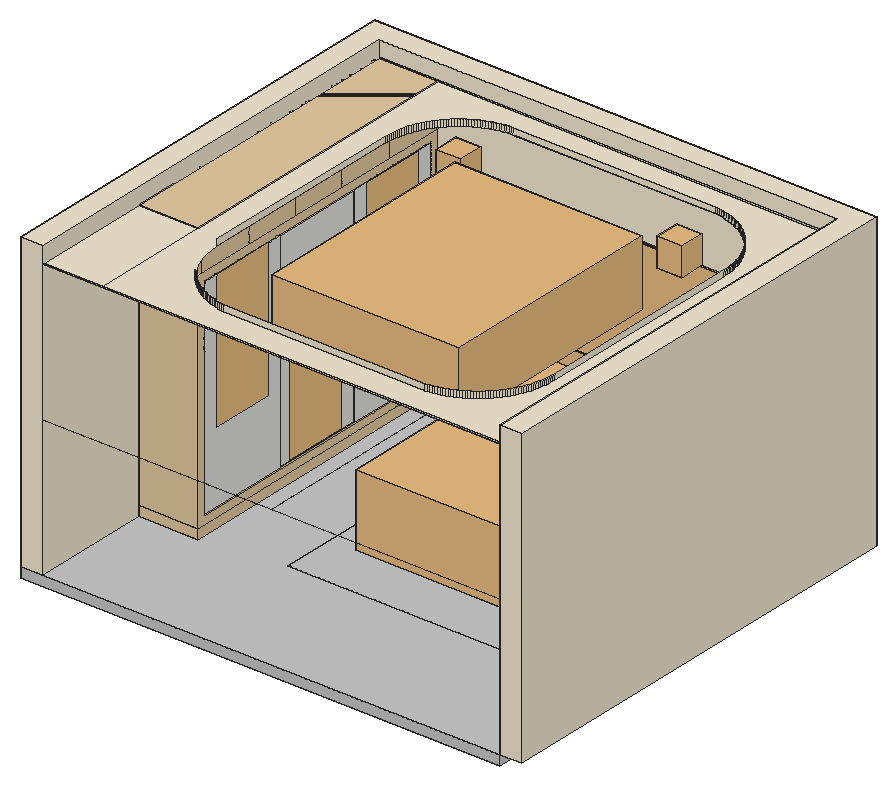
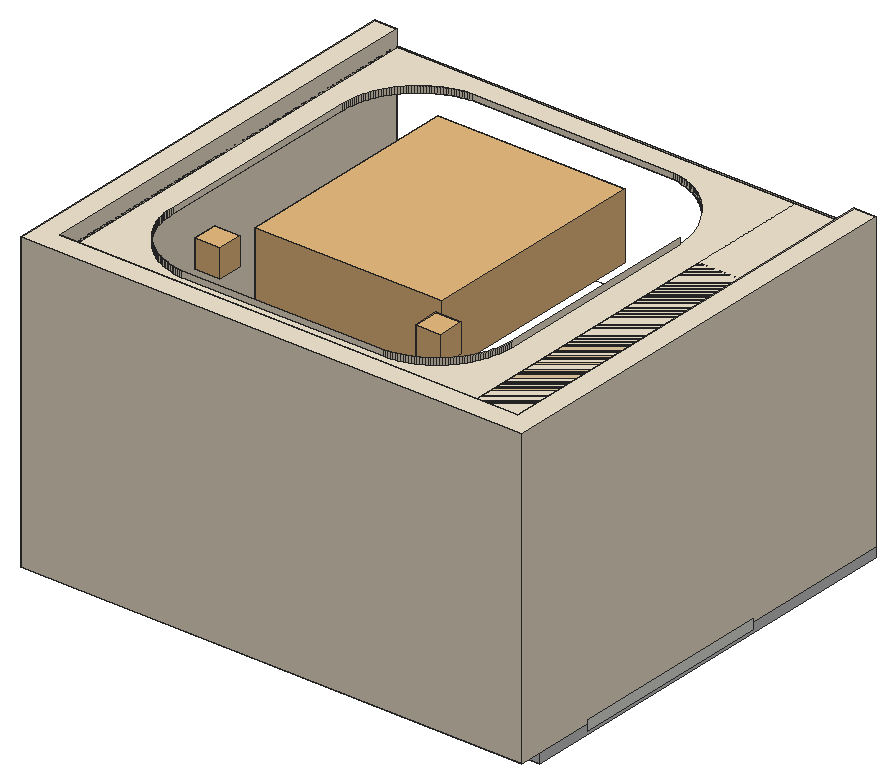
# SketchUp Ruby script. Lengths in inches.
U = 1.inch
M = Sketchup.active_model
def pt(a) = Geom::Point3d.new(a.map { |v| v * U })
def face(e, loops, mat)
  f = e.add_face(loops[0].map { |a| pt(a) })
  loops[1..].each { |l| e.add_face(l.map { |a| pt(a) }).erase! }
  f.material = f.back_material = mat if mat
  f
end
# faces: each face lists its corners as indices into pts; further lists are holes
def faces(e, pts, list, mat = nil) = list.each { |f| face(e, (f[0].is_a?(Array) ? f : [f]).map { |l| l.map { |i| pts[i] } }, mat) }
# xy, xz, yz: faces in a plane at the given z, y or x. An outline is a flat list of corners, or four numbers for a rectangle; further outlines are holes
def ring(l) = l.size == 4 ? [[l[0], l[1]], [l[2], l[1]], [l[2], l[3]], [l[0], l[3]]] : l.each_slice(2).to_a
def flat(e, list, mat, &to3) = list.each { |f| face(e, (f[0].is_a?(Array) ? f : [f]).map { |l| ring(l).map { |u, v| to3.(u, v) } }, mat) }
def xy(e, z, list, mat = nil) = flat(e, list, mat) { |x, y| [x, y, z] }
def xz(e, y, list, mat = nil) = flat(e, list, mat) { |x, z| [x, y, z] }
def yz(e, x, list, mat = nil) = flat(e, list, mat) { |y, z| [x, y, z] }
def lines(e, pts, list) = list.each { |a, b| e.add_line(pt(pts[a]), pt(pts[b])) }
# prism: a flat outline (further loops are holes) pulled along v
def prism(e, loops, v, mat = nil)
  f = face(e, loops, mat); d = Geom::Vector3d.new(v.map { |x| x * U })
  f.pushpull(f.normal.samedirection?(d) ? d.length : -d.length)
end
def box(e, o, s, mat = nil) = prism(e, [[o, [o[0] + s[0], o[1], o[2]], [o[0] + s[0], o[1] + s[1], o[2]], [o[0], o[1] + s[1], o[2]]]], [0, 0, s[2]], mat)
def at(x, y, z, deg = 0) = Geom::Transformation.translation(pt([x, y, z])) * Geom::Transformation.rotation(ORIGIN, Z_AXIS, deg.degrees)
def axes(o, x, y, z) = Geom::Transformation.new([*x, 0, *y, 0, *z, 0, *pt(o).to_a, 1])
def part(name) = M.definitions.add(name)
# library, detail: a bought-in or finely detailed component or shape, given as its bounding box
def library(name, o, s) = part(name).tap { |d| box(d.entities, o, s) }
def detail(e, o, s) = box(e.add_group.entities, o, s)
def put(e, d, t, mat = nil) = e.add_instance(d, t).tap { |i| i.material = mat if mat }
def group(e, t, mat = nil) = e.add_group.tap { |g| g.transformation = t; g.material = mat if mat }.entities
root = M.entities
M.materials.add("0961 AP 7892 PALE IVORY").color = [243, 232, 209]
M.materials.add("0962 AP 9878 Bamboo Straw-N").color = [228, 203, 161]
M.materials.add("Acquerello Marble (TJ07TT)").color = [202, 201, 200]
M.materials.add("Generic").color = [255, 255, 255]
M.materials.add("Kit Kat Speckle_ Stack (OYOLJ5)").color = [227, 224, 217]
M.materials.add("The Belden Brick Company Dapple Gray Matt None Modular (3-5-").color = [200, 200, 200]
c1 = library("ceiling fan",[0,0,0],[76.25,93.13,30.02])
c2 = part("fan")
p = [[217.527,-902.72,540.318],[217.529,-902.72,540.318],[217.529,-902.72,541.354],[217.527,-902.72,541.354]]
lines(c2.entities,p,[[0,1],[2,3]])
put(c2.entities,c1,at(256.45,-350.9,679.41))
c3 = library("Side Table",[0,-0.77,-1.18],[23.62,18.49,23.93])
c4 = library("Group\#4",[-0.5,-1.92,0],[127,2.42,36])
c5 = library("Group\#18",[-0.5,-0.5,0],[151,1.71,48])
c6 = part("Group105\#1")
p = [[0,0,0],[0,0,-46.23],[-14.28,0,-46.23],[93,-56.66,0],[-93,-56.66,0],[93,56.66,0],
  [93,0,0],[-93,56.66,0],[14.28,0,-46.23],[-93,0,0],[0,0,-74.83]]
lines(c6.entities,p,[[0,1],[1,2],[3,4],[5,6],[7,5],[1,8],[9,0],[0,6],[8,10],[4,9],[6,3],[2,10],
  [9,7]])
c7 = part("Rectangle Light\#1")
put(c7.entities,c6,at(0,0,0))
c8 = library("Bed 001",[-37.84,-46.07,0],[75.19,90.39,37.01])
c9 = library("Group\#5",[-0.5,-0.74,0],[30,1.24,80])
c10 = part("Group8\#1")
xy(c10.entities,7,[[-26.93,80.42,-2.93,81.13],[-26.93,109.26,-2.93,109.97],[-26.93,138.1,-2.93,138.81]])
xy(c10.entities,42.65,[[-26.93,51.9375,-2.93,80.42],[-26.93,81.13,-2.93,109.26],[-26.93,109.97,-2.93,138.1],[-26.93,138.81,-2.93,167.29]])
xy(c10.entities,43.35,[[-26.93,51.9375,-2.93,80.78],[-26.93,80.78,-2.93,109.26],[-26.93,109.97,-2.93,138.45],[-26.93,138.45,-2.93,167.29]])
xy(c10.entities,93,[[-26.93,109.26,-2.93,109.97]])
xz(c10.entities,51.9375,[[-26.93,42.65,-2.93,43.35]])
xz(c10.entities,80.42,[[-26.93,7,-2.93,42.65]])
xz(c10.entities,81.13,[[-26.93,7,-2.93,42.65]])
xz(c10.entities,109.26,[[-26.93,7,-2.93,42.65],[-26.93,43.35,-2.93,93]])
xz(c10.entities,109.97,[[-26.93,7,-2.93,42.65],[-26.93,43.35,-2.93,93]])
xz(c10.entities,138.1,[[-26.93,7,-2.93,42.65]])
xz(c10.entities,138.81,[[-26.93,7,-2.93,42.65]])
xz(c10.entities,167.29,[[-26.93,42.65,-2.93,43.35]])
yz(c10.entities,-26.93,[[80.42,7,80.42,42.65,80.78,43,81.13,42.65,81.13,7],[109.26,7,109.26,42.65,109.61,43,109.97,42.65,109.97,7],[138.1,7,138.1,42.65,138.45,43,138.81,42.65,138.81,7],[51.9375,42.65,51.9375,43.35,80.78,43.35,80.78,43,80.42,42.65],[81.13,42.65,80.78,43,80.78,43.35,109.26,43.35,109.61,43,109.26,42.65],
  [109.97,42.65,109.61,43,109.97,43.35,138.45,43.35,138.45,43,138.1,42.65],[138.81,42.65,138.45,43,138.45,43.35,167.29,43.35,167.29,42.65],[109.61,43,109.26,43.35,109.26,93,109.97,93,109.97,43.35]])
yz(c10.entities,-2.93,[[80.42,7,81.13,7,81.13,42.65,80.78,43,80.42,42.65],[109.26,7,109.97,7,109.97,42.65,109.61,43,109.26,42.65],[138.1,7,138.81,7,138.81,42.65,138.45,43,138.1,42.65],[51.9375,42.65,80.42,42.65,80.78,43,80.78,43.35,51.9375,43.35],[81.13,42.65,109.26,42.65,109.61,43,109.26,43.35,80.78,43.35,80.78,43],
  [109.97,42.65,138.1,42.65,138.45,43,138.45,43.35,109.97,43.35,109.61,43],[138.81,42.65,167.29,42.65,167.29,43.35,138.45,43.35,138.45,43],[109.61,43,109.97,43.35,109.97,93,109.26,93,109.26,43.35]])
c11 = part("Group\#11")
box(c11.entities,[0,0,0],[0.71,37.98,84.58])
c12 = part("Group\#21")
box(c12.entities,[0,0,-0.71],[23.77,15.3125,0.71])
c13 = part("Group16\#1")
xy(c13.entities,96,[[-26.22,74.37,-0.64,75.08],[-26.22,98.16,-2.22,98.87],[-26.22,121.95,-2.22,122.65],[-26.22,145.73,-2.22,146.44]])
xy(c13.entities,111.3125,[[-26.22,74.37,-0.64,75.08],[-26.22,98.16,-2.22,98.87],[-26.22,121.95,-2.22,122.65],[-26.22,145.73,-2.22,146.44]])
xz(c13.entities,74.37,[[-26.22,96,-0.64,111.3125]])
xz(c13.entities,75.08,[[-26.22,96,-0.64,111.3125]])
xz(c13.entities,98.16,[[-26.22,96,-2.22,111.3125]])
xz(c13.entities,98.87,[[-26.22,96,-2.22,111.3125]])
xz(c13.entities,121.95,[[-26.22,96,-2.22,111.3125]])
xz(c13.entities,122.65,[[-26.22,96,-2.22,111.3125]])
xz(c13.entities,145.73,[[-26.22,96,-2.22,111.3125]])
xz(c13.entities,146.44,[[-26.22,96,-2.22,111.3125]])
yz(c13.entities,-26.22,[[74.37,96,75.08,111.3125],[98.16,96,98.87,111.3125],[121.95,96,122.65,111.3125],[145.73,96,146.44,111.3125]])
yz(c13.entities,-2.22,[[98.16,96,98.87,111.3125],[121.95,96,122.65,111.3125],[145.73,96,146.44,111.3125]])
yz(c13.entities,-0.64,[[74.37,96,75.08,111.3125]])
c14 = library("plafonjera+p5",[99.06,48.1875,1.61],[10.2,10.2,11.38])
xy(root,7,[[12.07,51.9375,34.66,138.45],[34.66,51.9375,36.07,51.9375,36.07,167.29,35.36,167.29,35.36,138.45,34.66,138.45],[12.07,138.45,34.66,167.29],[34.66,138.45,35.36,167.29]])
xy(root,7.71,[[34.66,52.65,35.36,166.58]])
xy(root,7.71,[[35.36,52.65,36.07,166.58]],"0962 AP 9878 Bamboo Straw-N")
xy(root,43,[[12.07,138.45,35.36,167.29]])
xy(root,92.29,[[34.66,52.65,35.36,166.58],[35.36,52.65,36.07,166.58]])
xy(root,93,[[12.07,51.9375,34.66,167.29],[34.66,51.9375,36.07,167.29]])
xy(root,96,[[12.07,48.9375,36.07,170.29]])
xy(root,113.3125,[[12,0,36,171],[[36,0,198,171],[76.2,12,158,12,158.91,12.1,159.8125,12.23,160.71,12.39,161.61,12.57,162.5,12.78,163.38,13.02,164.26,13.28,165.13,13.57,165.99,13.88,166.84,14.22,167.68,14.58,168.51,14.97,169.32,15.38,170.13,15.82,170.92,16.28,171.7,16.76,172.46,17.27,173.21,17.79,173.9375,18.34,174.65,18.91,175.35,19.5,176.03,20.11,176.69,20.74,177.34,21.39,177.96,22.0625,178.5625,22.75,179.15,23.45,179.71,24.18,180.25,24.91,180.77,25.67,181.27,26.43,181.74,27.22,182.19,28.01,182.62,28.82,183.02,29.64,183.4,30.47,183.75,31.32,184.08,32.17,184.39,33.03,184.66,33.91,184.92,34.78,185.14,35.67,185.34,36.5625,185.52,37.46,185.66,38.36,185.78,39.27,185.88,40.18,185.95,41.09,185.99,42.01,186,42.92,186,129,185.99,129.9,185.95,130.81,185.88,131.71,185.78,132.6,185.66,133.5,185.51,134.39,185.34,135.28,185.14,136.16,184.91,137.03,184.65,137.9,184.375,138.76,184.07,139.61,183.74,140.45,183.38,141.28,183,142.1,182.59,142.9,182.16,143.7,181.71,144.48,181.23,145.25,180.73,146,180.21,146.74,179.67,147.46,179.1,148.16,178.52,148.85,177.91,149.52,177.29,150.17,176.64,150.8,175.98,151.41,175.29,152.01,174.59,152.58,173.88,153.125,173.15,153.65,172.4,154.16,171.63,154.64,170.86,155.1,170.07,155.54,169.26,155.95,168.45,156.34,167.62,156.71,166.78,157.04,165.9375,157.36,165.08,157.65,164.22,157.91,163.34,158.14,162.47,158.35,161.58,158.54,160.69,158.69,159.8,158.82,158.9,158.92,158,159,76.2,159,75.3,158.93,74.39,158.83,73.5,158.71,72.6,158.56,71.71,158.38,70.83,158.17,69.95,157.94,69.08,157.6875,68.22,157.4,67.37,157.09,66.52,156.76,65.69,156.4,64.87,156.01,64.0625,155.6,63.27,155.17,62.48,154.71,61.71,154.23,60.96,153.72,60.22,153.19,59.5,152.64,58.8,152.07,58.11,151.48,57.4375,150.87,56.79,150.24,56.16,149.59,55.55,148.92,54.96,148.23,54.39,147.52,53.84,146.8,53.3125,146.06,52.81,145.31,52.33,144.54,51.87,143.75,51.4375,142.96,51.03,142.15,50.64,141.32,50.28,140.49,49.95,139.65,49.64,138.8,49.36,137.93,49.1,137.0625,48.875,136.1875,48.67,135.3,48.49,134.41,48.34,133.52,48.22,132.62,48.125,131.72,48.06,130.8125,48.01,129.91,48,129,48,43.85,48.01,42.92,48.06,41.99,48.12,41.0625,48.22,40.14,48.34,39.22,48.49,38.3,48.66,37.38,48.86,36.48,49.09,35.57,49.34,34.68,49.62,33.79,49.92,32.91,50.25,32.04,50.61,31.18,50.99,30.33,51.39,29.5,51.82,28.67,52.27,27.86,52.75,27.06,53.24,26.27,53.76,25.5,54.31,24.75,54.87,24.01,55.46,23.29,56.0625,22.58,56.69,21.89,57.34,21.22,58,20.57,58.6875,19.94,59.39,19.33,60.11,18.74,60.84,18.18,61.6,17.63,62.36,17.1,63.15,16.6,63.94,16.12,64.75,15.67,65.58,15.23,66.41,14.82,67.26,14.44,68.12,14.08,68.98,13.75,69.86,13.4375,70.75,13.15,71.64,12.9,72.54,12.66,73.45,12.46,74.36,12.28,75.28,12.125]]],"0961 AP 7892 PALE IVORY")
xz(root,0,[[12,113.3125,198,113.78]],"0961 AP 7892 PALE IVORY")
xz(root,12,[[76.2,113.3125,158,115.78]],"0961 AP 7892 PALE IVORY")
xz(root,48.9375,[[12.07,4,36.07,96]],"0962 AP 9878 Bamboo Straw-N")
xz(root,51.9375,[[12.07,7,34.66,93],[34.66,7,36.07,93]])
xz(root,52.65,[[34.66,7.71,35.36,92.29],[35.36,7.71,36.07,92.29]])
xz(root,138.45,[[12.07,7,35.36,43]])
xz(root,159,[[76.2,113.3125,158,115.78]],"0961 AP 7892 PALE IVORY")
xz(root,166.58,[[34.66,7.71,35.36,92.29],[35.36,7.71,36.07,92.29]])
xz(root,167.29,[[12.07,7,34.66,43],[34.66,7,35.36,43],[35.36,7,36.07,7,36.07,93,34.66,93,34.66,43,35.36,43],[12.07,43,34.66,93]])
xz(root,170.29,[[12.07,4,36.07,96]])
xz(root,171,[[12,113.3125,198,113.78]],"0961 AP 7892 PALE IVORY")
yz(root,12,[[0,113.3125,171,113.78]],"0961 AP 7892 PALE IVORY")
yz(root,12.07,[[[48.9375,4,170.29,96],[51.9375,7,167.29,93]],[51.9375,7,80.78,43],[80.78,7,109.61,43],[109.61,7,138.45,43],[51.9375,43,109.61,93],
  [109.61,43,167.29,93]])
yz(root,34.66,[[[51.9375,7,167.29,93],[52.65,7.71,166.58,92.29]]])
yz(root,35.36,[[138.45,7,167.29,7,167.29,43,166.58,43,166.58,7.71,138.45,7.71],[138.45,7.71,166.58,43]])
yz(root,36.07,[[[48.9375,4,170.29,96],[51.9375,7,167.29,93]],[[51.9375,7,167.29,93],[52.65,7.71,166.58,92.29]]],"0962 AP 9878 Bamboo Straw-N")
yz(root,48,[[43.85,113.3125,129,115.78]],"0961 AP 7892 PALE IVORY")
yz(root,186,[[42.92,113.3125,129,115.78]],"0961 AP 7892 PALE IVORY")
yz(root,198,[[0,113.3125,171,113.78]],"0961 AP 7892 PALE IVORY")
p = [[76.2,12,113.3125],[75.28,12.125,113.3125],[75.28,12.125,115.78],[76.2,12,115.78],[158.91,12.1,113.3125],[158,12,113.3125],
  [158,12,115.78],[158.91,12.1,115.78],[74.36,12.28,113.3125],[74.36,12.28,115.78],[159.8125,12.23,113.3125],[159.8125,12.23,115.78],
  [160.71,12.39,113.3125],[160.71,12.39,115.78],[73.45,12.46,113.3125],[73.45,12.46,115.78],[161.61,12.57,113.3125],[161.61,12.57,115.78],
  [72.54,12.66,113.3125],[72.54,12.66,115.78],[162.5,12.78,113.3125],[162.5,12.78,115.78],[71.64,12.9,113.3125],[71.64,12.9,115.78],
  [163.38,13.02,113.3125],[163.38,13.02,115.78],[70.75,13.15,113.3125],[70.75,13.15,115.78],[164.26,13.28,113.3125],[164.26,13.28,115.78],
  [69.86,13.4375,113.3125],[69.86,13.4375,115.78],[165.13,13.57,113.3125],[165.13,13.57,115.78],[68.98,13.75,113.3125],[68.98,13.75,115.78],
  [165.99,13.88,113.3125],[165.99,13.88,115.78],[68.12,14.08,113.3125],[68.12,14.08,115.78],[166.84,14.22,113.3125],[166.84,14.22,115.78],
  [67.26,14.44,113.3125],[67.26,14.44,115.78],[167.68,14.58,113.3125],[167.68,14.58,115.78],[66.41,14.82,113.3125],[66.41,14.82,115.78],
  [168.51,14.97,113.3125],[168.51,14.97,115.78],[65.58,15.23,113.3125],[65.58,15.23,115.78],[169.32,15.38,113.3125],[169.32,15.38,115.78],
  [64.75,15.67,113.3125],[64.75,15.67,115.78],[170.13,15.82,113.3125],[170.13,15.82,115.78],[63.94,16.12,113.3125],[63.94,16.12,115.78],
  [170.92,16.28,113.3125],[170.92,16.28,115.78],[63.15,16.6,113.3125],[63.15,16.6,115.78],[171.7,16.76,113.3125],[171.7,16.76,115.78],
  [62.36,17.1,113.3125],[62.36,17.1,115.78],[172.46,17.27,113.3125],[172.46,17.27,115.78],[61.6,17.63,113.3125],[61.6,17.63,115.78],
  [173.21,17.79,113.3125],[173.21,17.79,115.78],[60.84,18.18,113.3125],[60.84,18.18,115.78],[173.9375,18.34,113.3125],[173.9375,18.34,115.78],
  [60.11,18.74,113.3125],[60.11,18.74,115.78],[174.65,18.91,113.3125],[174.65,18.91,115.78],[59.39,19.33,113.3125],[59.39,19.33,115.78],
  [175.35,19.5,113.3125],[175.35,19.5,115.78],[58.6875,19.94,113.3125],[58.6875,19.94,115.78],[176.03,20.11,113.3125],[176.03,20.11,115.78],
  [58,20.57,113.3125],[58,20.57,115.78],[176.69,20.74,113.3125],[176.69,20.74,115.78],[57.34,21.22,113.3125],[57.34,21.22,115.78],
  [177.34,21.39,113.3125],[177.34,21.39,115.78],[56.69,21.89,113.3125],[56.69,21.89,115.78],[177.96,22.0625,113.3125],[177.96,22.0625,115.78],
  [56.0625,22.58,113.3125],[56.0625,22.58,115.78],[178.5625,22.75,113.3125],[178.5625,22.75,115.78],[55.46,23.29,113.3125],[55.46,23.29,115.78],
  [179.15,23.45,113.3125],[179.15,23.45,115.78],[54.87,24.01,113.3125],[54.87,24.01,115.78],[179.71,24.18,113.3125],[179.71,24.18,115.78],
  [180.25,24.91,113.3125],[180.25,24.91,115.78],[180.77,25.67,113.3125],[180.77,25.67,115.78],[181.27,26.43,113.3125],[181.27,26.43,115.78],
  [181.74,27.22,113.3125],[181.74,27.22,115.78],[182.19,28.01,113.3125],[182.19,28.01,115.78],[182.62,28.82,113.3125],[182.62,28.82,115.78],
  [183.02,29.64,113.3125],[183.02,29.64,115.78],[183.4,30.47,113.3125],[183.4,30.47,115.78],[183.75,31.32,113.3125],[183.75,31.32,115.78],
  [184.08,32.17,113.3125],[184.08,32.17,115.78],[184.39,33.03,113.3125],[184.39,33.03,115.78],[184.66,33.91,113.3125],[184.66,33.91,115.78],
  [184.92,34.78,113.3125],[184.92,34.78,115.78],[185.14,35.67,113.3125],[185.14,35.67,115.78],[185.34,36.5625,113.3125],[185.34,36.5625,115.78],
  [185.52,37.46,113.3125],[185.52,37.46,115.78],[185.66,38.36,113.3125],[185.66,38.36,115.78],[185.78,39.27,113.3125],[185.78,39.27,115.78],
  [185.88,40.18,113.3125],[185.88,40.18,115.78],[185.95,41.09,113.3125],[185.95,41.09,115.78],[185.99,42.01,113.3125],[185.99,42.01,115.78],
  [186,42.92,113.3125],[186,42.92,115.78],[48,129,113.3125],[48.01,129.91,113.3125],[48.01,129.91,115.78],[48,129,115.78],
  [185.99,129.9,113.3125],[186,129,113.3125],[186,129,115.78],[185.99,129.9,115.78],[48.06,130.8125,113.3125],[48.06,130.8125,115.78],
  [185.95,130.81,113.3125],[185.95,130.81,115.78],[48.125,131.72,113.3125],[48.125,131.72,115.78],[185.88,131.71,113.3125],[185.88,131.71,115.78],
  [48.22,132.62,113.3125],[48.22,132.62,115.78],[185.78,132.6,113.3125],[185.78,132.6,115.78],[48.34,133.52,113.3125],[48.34,133.52,115.78],
  [185.66,133.5,113.3125],[185.66,133.5,115.78],[48.49,134.41,113.3125],[48.49,134.41,115.78],[185.51,134.39,113.3125],[185.51,134.39,115.78],
  [48.67,135.3,113.3125],[48.67,135.3,115.78],[185.34,135.28,113.3125],[185.34,135.28,115.78],[48.875,136.1875,113.3125],[48.875,136.1875,115.78],
  [185.14,136.16,113.3125],[185.14,136.16,115.78],[49.1,137.0625,113.3125],[49.1,137.0625,115.78],[184.91,137.03,113.3125],[184.91,137.03,115.78],
  [184.65,137.9,113.3125],[184.65,137.9,115.78],[49.36,137.93,113.3125],[49.36,137.93,115.78],[49.64,138.8,113.3125],[49.64,138.8,115.78],
  [184.375,138.76,113.3125],[184.375,138.76,115.78],[49.95,139.65,113.3125],[49.95,139.65,115.78],[184.07,139.61,113.3125],[184.07,139.61,115.78],
  [50.28,140.49,113.3125],[50.28,140.49,115.78],[183.74,140.45,113.3125],[183.74,140.45,115.78],[183.38,141.28,113.3125],[183.38,141.28,115.78],
  [50.64,141.32,113.3125],[50.64,141.32,115.78],[51.03,142.15,113.3125],[51.03,142.15,115.78],[183,142.1,113.3125],[183,142.1,115.78],
  [51.4375,142.96,113.3125],[51.4375,142.96,115.78],[182.59,142.9,113.3125],[182.59,142.9,115.78],[182.16,143.7,113.3125],[182.16,143.7,115.78],
  [51.87,143.75,113.3125],[51.87,143.75,115.78],[181.71,144.48,113.3125],[181.71,144.48,115.78],[52.33,144.54,113.3125],[52.33,144.54,115.78],
  [52.81,145.31,113.3125],[52.81,145.31,115.78],[181.23,145.25,113.3125],[181.23,145.25,115.78],[180.73,146,113.3125],[180.73,146,115.78],
  [53.3125,146.06,113.3125],[53.3125,146.06,115.78],[180.21,146.74,113.3125],[180.21,146.74,115.78],[53.84,146.8,113.3125],[53.84,146.8,115.78],
  [179.67,147.46,113.3125],[179.67,147.46,115.78],[54.39,147.52,113.3125],[54.39,147.52,115.78],[54.96,148.23,113.3125],[54.96,148.23,115.78],
  [179.1,148.16,113.3125],[179.1,148.16,115.78],[55.55,148.92,113.3125],[55.55,148.92,115.78],[178.52,148.85,113.3125],[178.52,148.85,115.78],
  [177.91,149.52,113.3125],[177.91,149.52,115.78],[56.16,149.59,113.3125],[56.16,149.59,115.78],[177.29,150.17,113.3125],[177.29,150.17,115.78],
  [56.79,150.24,113.3125],[56.79,150.24,115.78],[57.4375,150.87,113.3125],[57.4375,150.87,115.78],[176.64,150.8,113.3125],[176.64,150.8,115.78],
  [175.98,151.41,113.3125],[175.98,151.41,115.78],[58.11,151.48,113.3125],[58.11,151.48,115.78],[175.29,152.01,113.3125],[175.29,152.01,115.78],
  [58.8,152.07,113.3125],[58.8,152.07,115.78],[174.59,152.58,113.3125],[174.59,152.58,115.78],[59.5,152.64,113.3125],[59.5,152.64,115.78],
  [60.22,153.19,113.3125],[60.22,153.19,115.78],[173.88,153.125,113.3125],[173.88,153.125,115.78],[173.15,153.65,113.3125],[173.15,153.65,115.78],
  [60.96,153.72,113.3125],[60.96,153.72,115.78],[61.71,154.23,113.3125],[61.71,154.23,115.78],[172.4,154.16,113.3125],[172.4,154.16,115.78],
  [62.48,154.71,113.3125],[62.48,154.71,115.78],[171.63,154.64,113.3125],[171.63,154.64,115.78],[170.86,155.1,113.3125],[170.86,155.1,115.78],
  [63.27,155.17,113.3125],[63.27,155.17,115.78],[170.07,155.54,113.3125],[170.07,155.54,115.78],[64.0625,155.6,113.3125],[64.0625,155.6,115.78],
  [169.26,155.95,113.3125],[169.26,155.95,115.78],[64.87,156.01,113.3125],[64.87,156.01,115.78],[65.69,156.4,113.3125],[65.69,156.4,115.78],
  [168.45,156.34,113.3125],[168.45,156.34,115.78],[167.62,156.71,113.3125],[167.62,156.71,115.78],[66.52,156.76,113.3125],[66.52,156.76,115.78],
  [166.78,157.04,113.3125],[166.78,157.04,115.78],[67.37,157.09,113.3125],[67.37,157.09,115.78],[165.9375,157.36,113.3125],[165.9375,157.36,115.78],
  [68.22,157.4,113.3125],[68.22,157.4,115.78],[69.08,157.6875,113.3125],[69.08,157.6875,115.78],[165.08,157.65,113.3125],[165.08,157.65,115.78],
  [164.22,157.91,113.3125],[164.22,157.91,115.78],[69.95,157.94,113.3125],[69.95,157.94,115.78],[70.83,158.17,113.3125],[70.83,158.17,115.78],
  [163.34,158.14,113.3125],[163.34,158.14,115.78],[162.47,158.35,113.3125],[162.47,158.35,115.78],[71.71,158.38,113.3125],[71.71,158.38,115.78],
  [72.6,158.56,113.3125],[72.6,158.56,115.78],[161.58,158.54,113.3125],[161.58,158.54,115.78],[160.69,158.69,113.3125],[160.69,158.69,115.78],
  [73.5,158.71,113.3125],[73.5,158.71,115.78],[74.39,158.83,113.3125],[74.39,158.83,115.78],[159.8,158.82,113.3125],[159.8,158.82,115.78],
  [75.3,158.93,113.3125],[75.3,158.93,115.78],[158.9,158.92,113.3125],[158.9,158.92,115.78],[76.2,159,113.3125],[76.2,159,115.78],
  [158,159,113.3125],[158,159,115.78],[36,171.01,113.3125],[36,171,113.3125]]
faces(root,p,[[0,1,2,3],[4,5,6,7],[1,8,9,2],[10,4,7,11],[12,10,11,13],[8,14,15,9],[16,12,13,17],[14,18,19,15],
  [20,16,17,21],[18,22,23,19],[24,20,21,25],[22,26,27,23],[28,24,25,29],[26,30,31,27],[32,28,29,33],[30,34,35,31],
  [36,32,33,37],[34,38,39,35],[40,36,37,41],[38,42,43,39],[44,40,41,45],[42,46,47,43],[48,44,45,49],[46,50,51,47],
  [52,48,49,53],[50,54,55,51],[56,52,53,57],[54,58,59,55],[60,56,57,61],[58,62,63,59],[64,60,61,65],[62,66,67,63],
  [68,64,65,69],[66,70,71,67],[72,68,69,73],[70,74,75,71],[76,72,73,77],[74,78,79,75],[80,76,77,81],[78,82,83,79],
  [84,80,81,85],[82,86,87,83],[88,84,85,89],[86,90,91,87],[92,88,89,93],[90,94,95,91],[96,92,93,97],[94,98,99,95],
  [100,96,97,101],[98,102,103,99],[104,100,101,105],[102,106,107,103],[108,104,105,109],[106,110,111,107],[112,108,109,113],[114,112,113,115],
  [116,114,115,117],[118,116,117,119],[120,118,119,121],[122,120,121,123],[124,122,123,125],[126,124,125,127],[128,126,127,129],[130,128,129,131],
  [132,130,131,133],[134,132,133,135],[136,134,135,137],[138,136,137,139],[140,138,139,141],[142,140,141,143],[144,142,143,145],[146,144,145,147],
  [148,146,147,149],[150,148,149,151],[152,150,151,153],[154,152,153,155],[156,154,155,157],[158,159,160,161],[162,163,164,165],[159,166,167,160],
  [168,162,165,169],[166,170,171,167],[172,168,169,173],[170,174,175,171],[176,172,173,177],[174,178,179,175],[180,176,177,181],[178,182,183,179],
  [184,180,181,185],[182,186,187,183],[188,184,185,189],[186,190,191,187],[192,188,189,193],[190,194,195,191],[196,192,193,197],[198,196,197,199],
  [194,200,201,195],[200,202,203,201],[204,198,199,205],[202,206,207,203],[208,204,205,209],[206,210,211,207],[212,208,209,213],[214,212,213,215],
  [210,216,217,211],[216,218,219,217],[220,214,215,221],[218,222,223,219],[224,220,221,225],[226,224,225,227],[222,228,229,223],[230,226,227,231],
  [228,232,233,229],[232,234,235,233],[236,230,231,237],[238,236,237,239],[234,240,241,235],[242,238,239,243],[240,244,245,241],[246,242,243,247],
  [244,248,249,245],[248,250,251,249],[252,246,247,253],[250,254,255,251],[256,252,253,257],[258,256,257,259],[254,260,261,255],[262,258,259,263],
  [260,264,265,261],[264,266,267,265],[268,262,263,269],[270,268,269,271],[266,272,273,267],[274,270,271,275],[272,276,277,273],[278,274,275,279],
  [276,280,281,277],[280,282,283,281],[284,278,279,285],[286,284,285,287],[282,288,289,283],[288,290,291,289],[292,286,287,293],[290,294,295,291],
  [296,292,293,297],[298,296,297,299],[294,300,301,295],[302,298,299,303],[300,304,305,301],[306,302,303,307],[304,308,309,305],[308,310,311,309],
  [312,306,307,313],[314,312,313,315],[310,316,317,311],[318,314,315,319],[316,320,321,317],[322,318,319,323],[320,324,325,321],[324,326,327,325],
  [328,322,323,329],[330,328,329,331],[326,332,333,327],[332,334,335,333],[336,330,331,337],[338,336,337,339],[334,340,341,335],[340,342,343,341],
  [344,338,339,345],[346,344,345,347],[342,348,349,343],[348,350,351,349],[352,346,347,353],[350,354,355,351],[356,352,353,357],[354,358,359,355],
  [360,356,357,361]],"0961 AP 7892 PALE IVORY")
lines(root,p,[[362,363]])
put(root,c2,axes([-177.96,384.15,-516.08],[1,0,0],[0,1,0],[0,0,0.89415]))
g1 = group(root,at(36,0,0),"Acquerello Marble (TJ07TT)")
box(g1,[-33,0,-4],[195,171,4])
put(root,c3,axes([166.76,149.48,0],[1.3224,0,0],[0,1.21,0],[0,0,0.6966]))
g2 = group(root,at(27,0,0),"0961 AP 7892 PALE IVORY")
xy(g2,0,[[-24,0,-24,180,180,180,180,0,171,0,171,171,9,171,9,170.29,-15,170.29,-15,0],[9,170.29,45,171]])
xy(g2,36,[[74.51,170.29,135,171]])
xy(g2,120,[[-24,0,-15,0,-15,171,171,171,171,0,180,0,180,180,-24,180]])
xz(g2,0,[[-24,0,-15,120],[171,0,180,120]])
xz(g2,170.29,[[-15,0,45,0,45,11.29,45.81,14.67,47.01,17.94,48.57,21.05,50.49,23.96,52.73,26.62,55.26,29.01,58.06,31.08,61.07,32.82,64.27,34.2,67.61,35.19,71.03,35.8,74.51,36,135,36,135,48.98,134.27,53.67,132.97,58.24,131.12,62.62,128.75,66.73,125.89,70.52,122.58,73.93,118.88,76.91,114.84,79.41,110.53,81.39,106,82.83,101.33,83.71,96.59,84,-15,84]],"Kit Kat Speckle_ Stack (OYOLJ5)")
xz(g2,171,[[9,0,9,84,96.59,84,101.33,83.71,106,82.83,110.53,81.39,114.84,79.41,118.88,76.91,122.58,73.93,125.89,70.52,128.75,66.73,131.12,62.62,132.97,58.24,134.27,53.67,135,48.98,135,36,74.51,36,71.03,35.8,67.61,35.19,64.27,34.2,61.07,32.82,58.06,31.08,55.26,29.01,52.73,26.62,50.49,23.96,48.57,21.05,47.01,17.94,45.81,14.67,45,11.29,45,0],[135,36,171,36,171,120,-15,120,-15,84,96.59,84,101.33,83.71,106,82.83,110.53,81.39,114.84,79.41,118.88,76.91,122.58,73.93,125.89,70.52,128.75,66.73,131.12,62.62,132.97,58.24,134.27,53.67,135,48.98]])
xz(g2,180,[[-24,0,180,120]])
yz(g2,-24,[[0,0,180,120]])
yz(g2,-15,[[0,0,170.29,0,170.29,84,171,84,171,120,0,120]])
yz(g2,45,[[170.29,0,171,11.29]])
yz(g2,171,[[0,0,171,120]])
yz(g2,180,[[0,0,180,120]])
p = [[45,171,11.29],[45.81,171,14.67],[45.81,170.29,14.67],[45,170.29,11.29],[47.01,171,17.94],[47.01,170.29,17.94],
  [48.57,171,21.05],[48.57,170.29,21.05],[50.49,171,23.96],[50.49,170.29,23.96],[52.73,171,26.62],[52.73,170.29,26.62],
  [55.26,171,29.01],[55.26,170.29,29.01],[58.06,171,31.08],[58.06,170.29,31.08],[61.07,171,32.82],[61.07,170.29,32.82],
  [64.27,171,34.2],[64.27,170.29,34.2],[67.61,171,35.19],[67.61,170.29,35.19],[71.03,171,35.8],[71.03,170.29,35.8],
  [74.51,171,36],[74.51,170.29,36],[135,171,0],[135,171,-0.0625]]
faces(g2,p,[[0,1,2,3],[1,4,5,2],[4,6,7,5],[6,8,9,7],[8,10,11,9],[10,12,13,11],[12,14,15,13],[14,16,17,15],
  [16,18,19,17],[18,20,21,19],[20,22,23,21],[22,24,25,23]])
lines(g2,p,[[26,27]])
put(g2,c4,at(45,171,0))
put(g2,c5,at(-15,170.29,36))
put(root,c7,axes([105,-0.01,56.66],[1,0,0],[0,0,-1],[0,-1.78143,0]))
g3 = group(root,at(0,66.51,0))
yz(g3,0,[[0,0,84.09,4]])
g4 = group(root,at(12.07,66.51,4),"0962 AP 9878 Bamboo Straw-N")
box(g4,[0,-17.57,-4],[24,121.35,4])
g5 = group(root,at(63.27,29.25,0),"The Belden Brick Company Dapple Gray Matt None Modular (3-5-")
box(g5,[6,24,0],[91,84,0.24])
put(root,c8,axes([119.04,123.37,0.24],[1.04,0,0],[0,1.06,0],[0,0,0.79]))
put(root,c9,at(38,170.29,1.5),"Generic")
put(root,c10,at(37.58,0,0))
g6 = group(root,at(35.36,52.65,7.71))
box(g6,[0,0,0],[0.71,37.98,84.58])
g7 = group(root,at(34.66,122.6,63.28),"0962 AP 9878 Bamboo Straw-N")
detail(g7,[0,-25.98,-55.57],[0.75,25.98,55.57])
put(root,c11,axes([34.66,128.6,92.29],[1,0,0],[0,-1,0],[0,0,-1]))
put(root,c11,at(35.36,128.6,7.71))
g8 = group(root,at(35.36,58.65,36.72),"0962 AP 9878 Bamboo Straw-N")
detail(g8,[0,0,0],[0.75,25.98,55.57])
g9 = group(root,at(35.36,134.6,36.72),"0962 AP 9878 Bamboo Straw-N")
detail(g9,[0,0,0],[0.75,25.98,55.57])
put(root,c12,axes([36.07,98.5,96],[0,1,0],[0,0,1],[1,0,0]),"0962 AP 9878 Bamboo Straw-N")
put(root,c12,axes([36.07,122.27,96],[0,1,0],[0,0,1],[1,0,0]),"0962 AP 9878 Bamboo Straw-N")
put(root,c12,axes([36.07,146.05,96],[0,1,0],[0,0,1],[1,0,0]),"0962 AP 9878 Bamboo Straw-N")
g10 = group(root,at(36.07,74.72,96),"0962 AP 9878 Bamboo Straw-N")
box(g10,[-0.71,0.08,0],[0.71,23.69,15.3125])
g11 = group(root,at(36.07,50.95,96),"0962 AP 9878 Bamboo Straw-N")
box(g11,[-0.71,0,0],[0.71,23.69,15.3125])
put(root,c13,at(36,0,0))
g12 = group(root,at(12,48.9375,96),"0962 AP 9878 Bamboo Straw-N")
xy(g12,0,[[0.01,0,-0.06,122.0625,24,122.08,24,120.08,0.71,120.0625,0.78,2,24.07,2.01,24.07,0.01]])
xy(g12,15.3125,[[0.78,2,0.71,120.0625,24,120.08,24.07,2.01]])
xy(g12,17.3125,[[0.01,0,24.07,0.01,24,122.08,-0.06,122.0625]])
p = [[-0.06,122.0625,0],[0.01,0,0],[0.01,0,17.3125],[-0.06,122.0625,17.3125],[24.07,0.01,0],[24.07,0.01,17.3125],
  [24,120.08,15.3125],[24,120.08,0],[24,122.08,0],[24,122.08,17.3125],[24.07,2.01,0],[24.07,2.01,15.3125],
  [0.78,2,15.3125],[0.78,2,0],[0.71,120.0625,0],[0.71,120.0625,15.3125],[0.78,25.79,15.3125],[0.78,25.79,0],
  [0.78,49.58,15.3125],[0.78,49.58,0],[0.78,73.36,15.3125],[0.78,73.36,0],[0.78,97.15,15.3125],[0.78,97.15,0],
  [0.78,120.9375,15.3125],[0.78,120.9375,0]]
faces(g12,p,[[0,1,2,3],[1,4,5,2],[6,7,8,9,5,4,10,11],[12,13,14,15],[13,12,11,10],[15,14,7,6],[3,9,8,0]])
lines(g12,p,[[16,17],[18,19],[20,21],[22,23],[24,25]])
put(root,c14,at(-32.13,82.95,103.79))
put(root,c14,at(57.87,82.95,103.79))
